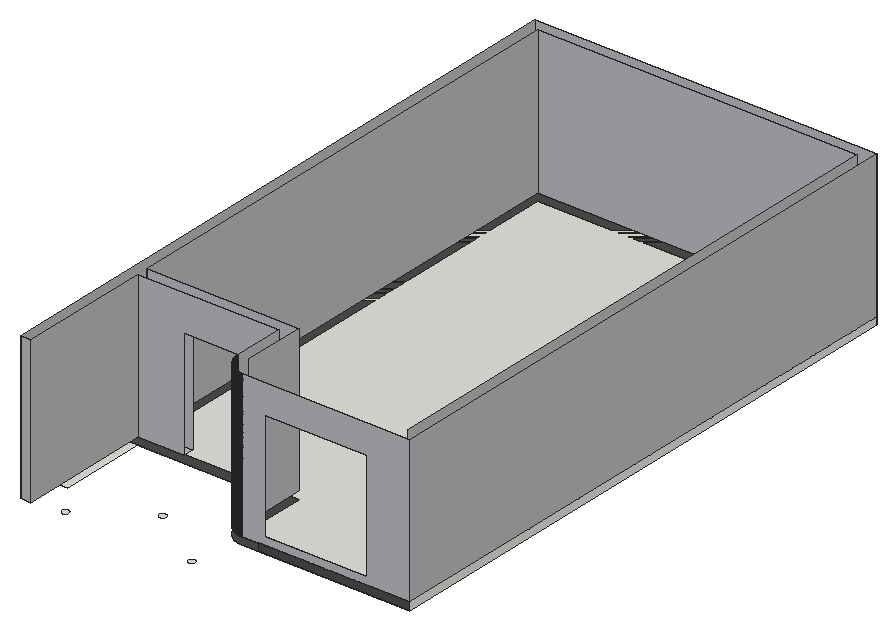
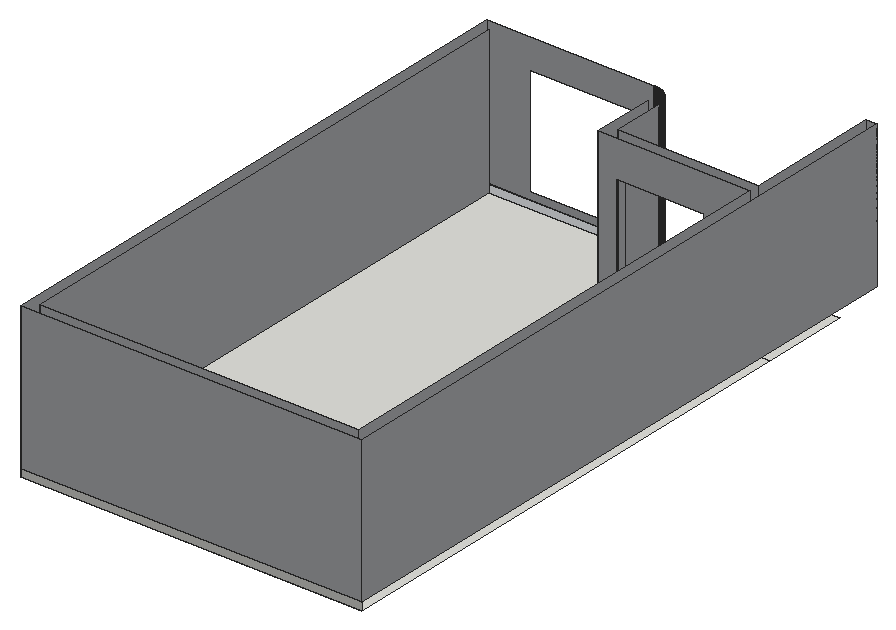
# SketchUp Ruby script. Lengths in inches.
U = 1.inch
M = Sketchup.active_model
def pt(a) = Geom::Point3d.new(a.map { |v| v * U })
def face(e, loops, mat)
  f = e.add_face(loops[0].map { |a| pt(a) })
  loops[1..].each { |l| e.add_face(l.map { |a| pt(a) }).erase! }
  f.material = f.back_material = mat if mat
  f
end
# faces: each face lists its corners as indices into pts; further lists are holes
def faces(e, pts, list, mat = nil) = list.each { |f| face(e, (f[0].is_a?(Array) ? f : [f]).map { |l| l.map { |i| pts[i] } }, mat) }
# xy, xz, yz: faces in a plane at the given z, y or x. An outline is a flat list of corners, or four numbers for a rectangle; further outlines are holes
def ring(l) = l.size == 4 ? [[l[0], l[1]], [l[2], l[1]], [l[2], l[3]], [l[0], l[3]]] : l.each_slice(2).to_a
def flat(e, list, mat, &to3) = list.each { |f| face(e, (f[0].is_a?(Array) ? f : [f]).map { |l| ring(l).map { |u, v| to3.(u, v) } }, mat) }
def xy(e, z, list, mat = nil) = flat(e, list, mat) { |x, y| [x, y, z] }
def xz(e, y, list, mat = nil) = flat(e, list, mat) { |x, z| [x, y, z] }
def yz(e, x, list, mat = nil) = flat(e, list, mat) { |y, z| [x, y, z] }
def lines(e, pts, list) = list.each { |a, b| e.add_line(pt(pts[a]), pt(pts[b])) }
# prism: a flat outline (further loops are holes) pulled along v
def prism(e, loops, v, mat = nil)
  f = face(e, loops, mat); d = Geom::Vector3d.new(v.map { |x| x * U })
  f.pushpull(f.normal.samedirection?(d) ? d.length : -d.length)
end
def box(e, o, s, mat = nil) = prism(e, [[o, [o[0] + s[0], o[1], o[2]], [o[0] + s[0], o[1] + s[1], o[2]], [o[0], o[1] + s[1], o[2]]]], [0, 0, s[2]], mat)
def at(x, y, z, deg = 0) = Geom::Transformation.translation(pt([x, y, z])) * Geom::Transformation.rotation(ORIGIN, Z_AXIS, deg.degrees)
def axes(o, x, y, z) = Geom::Transformation.new([*x, 0, *y, 0, *z, 0, *pt(o).to_a, 1])
def part(name) = M.definitions.add(name)
# library, detail: a bought-in or finely detailed component or shape, given as its bounding box
def library(name, o, s) = part(name).tap { |d| box(d.entities, o, s) }
def detail(e, o, s) = box(e.add_group.entities, o, s)
def put(e, d, t, mat = nil) = e.add_instance(d, t).tap { |i| i.material = mat if mat }
def group(e, t, mat = nil) = e.add_group.tap { |g| g.transformation = t; g.material = mat if mat }.entities
root = M.entities
M.materials.add("1423 AP 8230 BENTONITE").color = [77, 75, 77]
M.materials.add("1427 AP 686 ARMOUR-N").color = [184, 186, 189]
xy(root,245,[[35,153.42,34.92,153.43,34.84,153.43,34.76,153.44,34.6875,153.44,34.61,153.46,34.45,153.48,34.38,153.5,34.3,153.52,34.23,153.55,34.15,153.57,34.01,153.63,33.9375,153.66,33.87,153.7,33.8,153.73,33.73,153.77,33.66,153.8125,33.59,153.86,33.53,153.9,33.29,154.1,33.18,154.21,33.07,154.33,33.02,154.39,32.98,154.45,32.93,154.52,32.89,154.58,32.77,154.79,32.68,155,32.65,155.08,32.62,155.15,32.6,155.23,32.58,155.3,32.54,155.46,32.53,155.53,32.52,155.61,32.51,155.6875,32.51,155.77,32.5,155.85,32.5,156,32.51,156.08,32.51,156.16,32.53,156.32,32.54,156.39,32.58,156.55,32.6,156.62,32.62,156.7,32.68,156.84,32.71,156.92,32.77,157.06,32.85,157.2,32.89,157.26,32.93,157.33,32.98,157.39,33.02,157.46,33.07,157.52,33.18,157.64,33.29,157.75,33.53,157.95,33.59,157.99,33.66,158.04,33.8,158.12,33.87,158.15,33.9375,158.1875,34.01,158.22,34.15,158.28,34.23,158.3,34.3,158.33,34.38,158.35,34.45,158.36,34.53,158.38,34.61,158.39,34.6875,158.4,34.76,158.41,34.84,158.42,35.16,158.42,35.24,158.41,35.3125,158.4,35.39,158.39,35.47,158.38,35.55,158.36,35.62,158.35,35.7,158.33,35.77,158.3,35.85,158.28,35.99,158.22,36.06,158.1875,36.14,158.15,36.2,158.12,36.34,158.04,36.41,157.99,36.47,157.95,36.71,157.75,36.82,157.64,36.93,157.52,36.98,157.46,37.02,157.39,37.07,157.33,37.11,157.26,37.15,157.2,37.23,157.06,37.29,156.92,37.32,156.84,37.38,156.7,37.4,156.62,37.42,156.55,37.46,156.39,37.47,156.32,37.5,156.08,37.5,155.77,37.49,155.6875,37.48,155.61,37.47,155.53,37.46,155.46,37.42,155.3,37.4,155.23,37.38,155.15,37.35,155.08,37.32,155,37.23,154.79,37.11,154.58,37.07,154.52,37.02,154.45,36.98,154.39,36.93,154.33,36.82,154.21,36.71,154.1,36.47,153.9,36.41,153.86,36.34,153.8125,36.27,153.77,36.2,153.73,36.06,153.66,35.85,153.57,35.77,153.55,35.7,153.52,35.62,153.5,35.55,153.48,35.39,153.46,35.3125,153.44,35.24,153.44,35.16,153.43,35.08,153.43],[139,153.42,138.92,153.43,138.84,153.43,138.76,153.44,138.6875,153.44,138.61,153.46,138.45,153.48,138.38,153.5,138.3,153.52,138.23,153.55,138.15,153.57,138.01,153.63,137.9375,153.66,137.87,153.7,137.8,153.73,137.73,153.77,137.66,153.8125,137.59,153.86,137.53,153.9,137.29,154.1,137.18,154.21,137.07,154.33,137.02,154.39,136.98,154.45,136.93,154.52,136.89,154.58,136.77,154.79,136.68,155,136.65,155.08,136.62,155.15,136.6,155.23,136.58,155.3,136.54,155.46,136.53,155.53,136.52,155.61,136.51,155.6875,136.5,155.77,136.5,156.08,136.53,156.32,136.54,156.39,136.58,156.55,136.6,156.62,136.62,156.7,136.68,156.84,136.71,156.92,136.77,157.06,136.85,157.2,136.89,157.26,136.93,157.33,136.98,157.39,137.02,157.46,137.07,157.52,137.18,157.64,137.29,157.75,137.53,157.95,137.59,157.99,137.66,158.04,137.8,158.12,137.87,158.15,137.9375,158.1875,138.01,158.22,138.15,158.28,138.23,158.3,138.3,158.33,138.38,158.35,138.45,158.36,138.53,158.38,138.61,158.39,138.6875,158.4,138.76,158.41,138.84,158.42,139.16,158.42,139.24,158.41,139.3125,158.4,139.39,158.39,139.47,158.38,139.55,158.36,139.62,158.35,139.7,158.33,139.77,158.3,139.85,158.28,139.99,158.22,140.0625,158.1875,140.13,158.15,140.2,158.12,140.34,158.04,140.41,157.99,140.47,157.95,140.71,157.75,140.82,157.64,140.93,157.52,140.98,157.46,141.02,157.39,141.07,157.33,141.11,157.26,141.15,157.2,141.23,157.06,141.29,156.92,141.32,156.84,141.38,156.7,141.4,156.62,141.42,156.55,141.46,156.39,141.47,156.32,141.5,156.08,141.5,155.77,141.49,155.6875,141.48,155.61,141.47,155.53,141.46,155.46,141.42,155.3,141.4,155.23,141.38,155.15,141.35,155.08,141.32,155,141.23,154.79,141.11,154.58,141.07,154.52,141.02,154.45,140.98,154.39,140.93,154.33,140.82,154.21,140.71,154.1,140.47,153.9,140.41,153.86,140.34,153.8125,140.27,153.77,140.2,153.73,140.13,153.7,140.0625,153.66,139.99,153.63,139.85,153.57,139.77,153.55,139.7,153.52,139.62,153.5,139.55,153.48,139.39,153.46,139.3125,153.44,139.24,153.44,139.16,153.43,139.08,153.43],[86.84,188.5,86.76,188.51,86.6875,188.52,86.61,188.53,86.53,188.54,86.45,188.56,86.38,188.58,86.3,188.6,86.23,188.62,86.15,188.65,86.01,188.71,85.9375,188.74,85.87,188.77,85.59,188.93,85.53,188.98,85.47,189.02,85.41,189.07,85.29,189.18,85.23,189.23,85.18,189.29,85.07,189.41,85.02,189.47,84.98,189.53,84.93,189.59,84.77,189.87,84.74,189.9375,84.71,190.01,84.65,190.15,84.62,190.23,84.6,190.3,84.58,190.38,84.56,190.45,84.54,190.53,84.53,190.61,84.52,190.6875,84.51,190.76,84.5,190.84,84.5,191.16,84.51,191.24,84.52,191.3125,84.53,191.39,84.54,191.47,84.56,191.55,84.58,191.62,84.6,191.7,84.62,191.77,84.65,191.85,84.71,191.99,84.74,192.0625,84.77,192.13,84.93,192.41,84.98,192.47,85.02,192.53,85.07,192.59,85.18,192.71,85.23,192.77,85.29,192.82,85.41,192.93,85.47,192.98,85.53,193.02,85.59,193.07,85.87,193.23,85.9375,193.26,86.01,193.29,86.15,193.35,86.23,193.38,86.3,193.4,86.38,193.42,86.45,193.44,86.53,193.46,86.61,193.47,86.6875,193.48,86.76,193.49,86.84,193.5,87.16,193.5,87.24,193.49,87.3125,193.48,87.39,193.47,87.47,193.46,87.55,193.44,87.62,193.42,87.7,193.4,87.77,193.38,87.85,193.35,87.99,193.29,88.0625,193.26,88.13,193.23,88.41,193.07,88.47,193.02,88.53,192.98,88.59,192.93,88.71,192.82,88.77,192.77,88.82,192.71,88.93,192.59,88.98,192.53,89.02,192.47,89.07,192.41,89.23,192.13,89.26,192.0625,89.29,191.99,89.35,191.85,89.38,191.77,89.4,191.7,89.42,191.62,89.44,191.55,89.46,191.47,89.47,191.39,89.48,191.3125,89.49,191.24,89.5,191.16,89.5,190.84,89.49,190.76,89.48,190.6875,89.47,190.61,89.46,190.53,89.44,190.45,89.42,190.38,89.4,190.3,89.38,190.23,89.35,190.15,89.29,190.01,89.26,189.9375,89.23,189.87,89.07,189.59,89.02,189.53,88.98,189.47,88.93,189.41,88.82,189.29,88.77,189.23,88.71,189.18,88.59,189.07,88.53,189.02,88.47,188.98,88.41,188.93,88.13,188.77,88.0625,188.74,87.99,188.71,87.85,188.65,87.77,188.62,87.7,188.6,87.62,188.58,87.55,188.56,87.47,188.54,87.39,188.53,87.3125,188.52,87.24,188.51,87.16,188.5]])
xy(root,246,[[9,180,18,252],[151.78,192,151.57,192.01,151.35,192.01,150.91,192.03,150.7,192.05,150.48,192.0625,150.26,192.08,150.05,192.11,149.83,192.13,149.61,192.16,149.4,192.1875,149.18,192.22,148.97,192.26,148.76,192.29,148.54,192.34,148.12,192.42,147.9,192.47,147.69,192.52,147.48,192.58,147.27,192.63,147.0625,192.69,146.85,192.75,146.64,192.81,146.4375,192.88,146.23,192.95,146.03,193.02,145.82,193.09,145.62,193.17,145.41,193.25,145.01,193.41,144.8125,193.5,144.61,193.59,144.41,193.68,144.22,193.77,144.02,193.86,143.83,193.96,143.63,194.0625,143.44,194.16,143.25,194.27,142.875,194.48,142.6875,194.6,142.5,194.71,142.32,194.83,142.14,194.94,141.95,195.0625,141.77,195.1875,141.6,195.3125,141.42,195.4375,141.24,195.57,140.9,195.83,140.73,195.97,140.56,196.1,140.39,196.24,140.23,196.38,140.0625,196.53,139.9,196.67,139.58,196.97,139.43,197.12,139.27,197.27,139.12,197.43,138.97,197.58,138.67,197.9,138.53,198.0625,138.38,198.23,138.24,198.39,138.1,198.56,137.97,198.73,137.83,198.9,137.57,199.24,137.4375,199.42,137.3125,199.6,137.1875,199.77,137.0625,199.95,136.94,200.14,136.83,200.32,136.71,200.5,136.6,200.6875,136.48,200.875,136.27,201.25,136.16,201.44,136.0625,201.63,135.96,201.83,135.86,202.02,135.77,202.22,135.68,202.41,135.59,202.61,135.5,202.8125,135.41,203.01,135.25,203.41,135.17,203.62,135.09,203.82,135.02,204.03,134.95,204.23,134.88,204.4375,134.81,204.64,134.75,204.85,134.69,205.0625,134.63,205.27,134.58,205.48,134.52,205.69,134.47,205.9,134.42,206.12,134.34,206.54,134.29,206.76,134.26,206.97,134.22,207.18,134.1875,207.4,134.16,207.61,134.13,207.83,134.11,208.05,134.08,208.26,134.0625,208.48,134.05,208.7,134.03,208.91,134.01,209.35,134.01,209.57,134,209.78,134,252,9,252,9,672,290,672,290,192]])
xy(root,246,[[[9,180,18,180,18,252,134,252,134,209.78,134.01,209.57,134.01,209.35,134.03,208.91,134.05,208.7,134.0625,208.48,134.08,208.26,134.11,208.05,134.13,207.83,134.16,207.61,134.1875,207.4,134.22,207.18,134.26,206.97,134.29,206.76,134.34,206.54,134.42,206.12,134.47,205.9,134.52,205.69,134.58,205.48,134.63,205.27,134.69,205.0625,134.75,204.85,134.82,204.64,134.88,204.4375,134.95,204.23,135.02,204.03,135.09,203.82,135.17,203.62,135.25,203.41,135.41,203.01,135.5,202.8125,135.59,202.61,135.68,202.41,135.77,202.22,135.86,202.02,135.96,201.83,136.0625,201.63,136.16,201.44,136.27,201.25,136.48,200.875,136.6,200.6875,136.71,200.5,136.83,200.32,136.94,200.14,137.0625,199.95,137.1875,199.77,137.3125,199.6,137.4375,199.42,137.57,199.24,137.83,198.9,137.97,198.73,138.1,198.56,138.24,198.39,138.38,198.23,138.53,198.0625,138.67,197.9,138.97,197.58,139.12,197.43,139.27,197.27,139.43,197.12,139.58,196.97,139.9,196.67,140.0625,196.53,140.23,196.38,140.39,196.24,140.56,196.1,140.73,195.97,140.9,195.83,141.24,195.57,141.42,195.4375,141.6,195.3125,141.77,195.1875,141.95,195.0625,142.14,194.94,142.32,194.83,142.5,194.71,142.6875,194.6,142.875,194.48,143.25,194.27,143.44,194.16,143.63,194.0625,143.83,193.96,144.02,193.86,144.22,193.77,144.41,193.68,144.61,193.59,144.8125,193.5,145.01,193.41,145.41,193.25,145.62,193.17,145.82,193.09,146.03,193.02,146.23,192.95,146.4375,192.88,146.64,192.82,146.85,192.75,147.0625,192.69,147.27,192.63,147.48,192.58,147.69,192.52,147.9,192.47,148.12,192.42,148.54,192.34,148.76,192.29,148.97,192.26,149.18,192.22,149.4,192.1875,149.61,192.16,149.83,192.13,150.05,192.11,150.26,192.08,150.48,192.0625,150.7,192.05,150.91,192.03,151.35,192.01,151.57,192.01,151.78,192,290,192,290,672,9,672],[151.78,201,151.67,201.01,151.57,201.01,151.46,201.02,151.35,201.02,151.02,201.05,150.92,201.07,150.7,201.09,150.48,201.13,150.38,201.15,150.27,201.17,150.16,201.1875,150.06,201.21,149.95,201.24,149.85,201.26,149.74,201.29,149.64,201.32,149.53,201.35,149.43,201.375,149.32,201.41,149.12,201.47,149.01,201.51,148.91,201.55,148.81,201.58,148.71,201.625,148.61,201.66,148.51,201.71,148.31,201.79,148.21,201.84,148.11,201.88,147.91,201.98,147.82,202.03,147.72,202.08,147.625,202.13,147.53,202.1875,147.4375,202.24,147.34,202.3,147.25,202.35,146.89,202.59,146.8,202.66,146.62,202.78,146.54,202.85,146.45,202.92,146.36,202.98,146.2,203.12,146.11,203.19,146.03,203.26,145.95,203.34,145.79,203.48,145.71,203.56,145.64,203.64,145.56,203.71,145.48,203.79,145.34,203.95,145.26,204.03,145.19,204.11,145.12,204.2,144.98,204.36,144.92,204.45,144.85,204.54,144.78,204.62,144.66,204.8,144.59,204.89,144.35,205.25,144.3,205.34,144.24,205.4375,144.1875,205.53,144.13,205.625,144.08,205.72,144.03,205.82,143.98,205.91,143.88,206.11,143.84,206.21,143.79,206.31,143.71,206.51,143.66,206.61,143.625,206.71,143.58,206.81,143.55,206.91,143.51,207.01,143.47,207.12,143.41,207.32,143.375,207.43,143.35,207.53,143.32,207.64,143.29,207.74,143.26,207.85,143.24,207.95,143.21,208.06,143.1875,208.16,143.17,208.27,143.15,208.38,143.13,208.48,143.09,208.7,143.07,208.92,143.05,209.02,143.02,209.35,143.02,209.46,143.01,209.57,143.01,209.67,143,209.78,143,261,18,261,18,663,281,663,281,201]]],"1423 AP 8230 BENTONITE")
xy(root,252,[[9,141.92,9,672,290,672,290,192,151.78,192,151.57,192.01,151.35,192.01,150.91,192.03,150.7,192.05,150.48,192.0625,150.26,192.08,150.05,192.11,149.83,192.13,149.61,192.16,149.4,192.1875,149.18,192.22,148.97,192.26,148.76,192.29,148.54,192.34,148.12,192.42,147.9,192.47,147.69,192.52,147.48,192.58,147.27,192.63,147.0625,192.69,146.85,192.75,146.64,192.82,146.4375,192.88,146.23,192.95,146.03,193.02,145.82,193.09,145.62,193.17,145.41,193.25,145.01,193.41,144.8125,193.5,144.61,193.59,144.41,193.68,144.22,193.77,144.02,193.86,143.83,193.96,143.63,194.0625,143.44,194.16,143.25,194.27,142.875,194.48,142.6875,194.6,142.5,194.71,142.32,194.83,142.14,194.94,141.95,195.0625,141.77,195.1875,141.6,195.3125,141.42,195.4375,141.24,195.57,140.9,195.83,140.73,195.97,140.56,196.1,140.39,196.24,140.23,196.38,140.0625,196.53,139.9,196.67,139.58,196.97,139.43,197.12,139.27,197.27,139.12,197.43,138.97,197.58,138.67,197.9,138.53,198.0625,138.38,198.23,138.24,198.39,138.1,198.56,137.97,198.73,137.83,198.9,137.57,199.24,137.4375,199.42,137.3125,199.6,137.1875,199.77,137.0625,199.95,136.94,200.14,136.83,200.32,136.71,200.5,136.6,200.6875,136.48,200.875,136.27,201.25,136.16,201.44,136.0625,201.63,135.96,201.83,135.86,202.02,135.77,202.22,135.68,202.41,135.59,202.61,135.5,202.8125,135.41,203.01,135.25,203.41,135.17,203.62,135.09,203.82,135.02,204.03,134.95,204.23,134.88,204.4375,134.82,204.64,134.75,204.85,134.69,205.0625,134.63,205.27,134.58,205.48,134.52,205.69,134.47,205.9,134.42,206.12,134.34,206.54,134.29,206.76,134.26,206.97,134.22,207.18,134.1875,207.4,134.16,207.61,134.13,207.83,134.11,208.05,134.08,208.26,134.0625,208.48,134.05,208.7,134.03,208.91,134.01,209.35,134.01,209.57,134,209.78,134,252,128,252,128,261,143,261,143,209.78,143.01,209.67,143.01,209.57,143.02,209.46,143.02,209.35,143.05,209.02,143.07,208.92,143.09,208.7,143.13,208.48,143.15,208.38,143.17,208.27,143.1875,208.16,143.21,208.06,143.24,207.95,143.26,207.85,143.29,207.74,143.32,207.64,143.35,207.53,143.375,207.43,143.41,207.32,143.47,207.12,143.51,207.01,143.55,206.91,143.58,206.81,143.625,206.71,143.66,206.61,143.71,206.51,143.79,206.31,143.84,206.21,143.88,206.11,143.98,205.91,144.03,205.82,144.08,205.72,144.13,205.625,144.1875,205.53,144.24,205.4375,144.3,205.34,144.35,205.25,144.59,204.89,144.66,204.8,144.78,204.62,144.85,204.54,144.92,204.45,144.98,204.36,145.12,204.2,145.19,204.11,145.26,204.03,145.34,203.95,145.48,203.79,145.56,203.71,145.64,203.64,145.71,203.56,145.79,203.48,145.95,203.34,146.03,203.26,146.11,203.19,146.2,203.12,146.36,202.98,146.45,202.92,146.54,202.85,146.62,202.78,146.8,202.66,146.89,202.59,147.25,202.35,147.34,202.3,147.4375,202.24,147.53,202.1875,147.625,202.13,147.72,202.08,147.82,202.03,147.91,201.98,148.11,201.88,148.21,201.84,148.31,201.79,148.51,201.71,148.61,201.66,148.71,201.625,148.81,201.58,148.91,201.55,149.01,201.51,149.12,201.47,149.32,201.41,149.43,201.375,149.53,201.35,149.64,201.32,149.74,201.29,149.85,201.26,149.95,201.24,150.06,201.21,150.16,201.1875,150.27,201.17,150.38,201.15,150.48,201.13,150.7,201.09,150.92,201.07,151.02,201.05,151.35,201.02,151.46,201.02,151.57,201.01,151.67,201.01,151.78,201,281,201,281,663,18,663,18,261,56,261,56,252,18,252,18,141.92]],"1427 AP 686 ARMOUR-N")
xz(root,141.92,[[9,252,18,372]],"1427 AP 686 ARMOUR-N")
xz(root,192,[[165,246,290,252]],"1423 AP 8230 BENTONITE")
xz(root,192,[[151.78,252,152,372],[[152,252,290,372],[170,258,254,348]]],"1427 AP 686 ARMOUR-N")
xz(root,192.01,[[151.35,252,151.57,372]],"1427 AP 686 ARMOUR-N")
xz(root,252,[[18,252,56,252,56,342,128,342,128,252,134,252,134,372,18,372]],"1427 AP 686 ARMOUR-N")
xz(root,261,[[18,252,18,372,143,372,143,252,128,252,128,342,56,342,56,252]],"1427 AP 686 ARMOUR-N")
xz(root,663,[[18,252,281,372]],"1427 AP 686 ARMOUR-N")
xz(root,672,[[9,246,290,252]])
xz(root,672,[[9,252,290,372]],"1427 AP 686 ARMOUR-N")
yz(root,9,[[141.92,252,672,372]],"1427 AP 686 ARMOUR-N")
yz(root,18,[[141.92,252,252,372],[261,252,663,372]],"1427 AP 686 ARMOUR-N")
yz(root,134,[[210,252,252,372]],"1427 AP 686 ARMOUR-N")
yz(root,143,[[209.89,252,261,372]],"1427 AP 686 ARMOUR-N")
yz(root,281,[[201,252,663,372]],"1427 AP 686 ARMOUR-N")
yz(root,290,[[192,246,672,252]])
yz(root,290,[[192,252,672,372]],"1427 AP 686 ARMOUR-N")
p = [[150.7,192.05,372],[150.48,192.0625,372],[150.48,192.0625,252],[150.7,192.05,252],[150.91,192.03,372],[150.91,192.03,252],
  [151.13,192.02,372],[151.13,192.02,252],[151.35,192.01,372],[151.35,192.01,252],[151.78,192,372],[151.57,192.01,372],
  [151.57,192.01,252],[151.78,192,252],[149.83,192.13,372],[149.61,192.16,372],[149.61,192.16,252],[149.83,192.13,252],
  [150.05,192.11,372],[150.05,192.11,252],[150.26,192.08,372],[150.26,192.08,252],[149.18,192.22,372],[148.97,192.26,372],
  [148.97,192.26,252],[149.18,192.22,252],[149.4,192.1875,372],[149.4,192.1875,252],[148.54,192.34,372],[148.33,192.38,372],
  [148.33,192.38,252],[148.54,192.34,252],[148.76,192.29,372],[148.76,192.29,252],[148.12,192.42,372],[147.9,192.47,372],
  [147.9,192.47,252],[148.12,192.42,252],[147.69,192.52,372],[147.48,192.58,372],[147.48,192.58,252],[147.69,192.52,252],
  [147.27,192.63,372],[147.0625,192.69,372],[147.0625,192.69,252],[147.27,192.63,252],[146.85,192.75,372],[146.85,192.75,252],
  [146.64,192.82,372],[146.4375,192.88,372],[146.4375,192.88,252],[146.64,192.82,252],[146.23,192.95,372],[146.03,193.02,372],
  [146.03,193.02,252],[146.23,192.95,252],[145.82,193.09,372],[145.82,193.09,252],[145.62,193.17,372],[145.62,193.17,252],
  [145.41,193.25,372],[145.21,193.33,372],[145.21,193.33,252],[145.41,193.25,252],[145.01,193.41,372],[145.01,193.41,252],
  [144.8125,193.5,372],[144.8125,193.5,252],[144.61,193.59,372],[144.61,193.59,252],[144.41,193.68,372],[144.41,193.68,252],
  [144.22,193.77,372],[144.22,193.77,252],[144.02,193.86,372],[144.02,193.86,252],[143.83,193.96,372],[143.83,193.96,252],
  [143.63,194.0625,372],[143.63,194.0625,252],[143.44,194.16,372],[143.44,194.16,252],[143.25,194.27,372],[143.25,194.27,252],
  [143.0625,194.375,372],[143.0625,194.375,252],[142.875,194.48,372],[142.875,194.48,252],[142.6875,194.6,372],[142.6875,194.6,252],
  [142.5,194.71,372],[142.5,194.71,252],[142.32,194.83,372],[142.32,194.83,252],[142.14,194.94,372],[142.14,194.94,252],
  [141.95,195.0625,372],[141.95,195.0625,252],[141.77,195.1875,372],[141.77,195.1875,252],[141.6,195.3125,372],[141.6,195.3125,252],
  [141.42,195.4375,372],[141.42,195.4375,252],[141.24,195.57,372],[141.24,195.57,252],[141.07,195.7,372],[141.07,195.7,252],
  [140.9,195.83,372],[140.9,195.83,252],[140.73,195.97,372],[140.73,195.97,252],[140.56,196.1,372],[140.56,196.1,252],
  [140.39,196.24,372],[140.39,196.24,252],[140.23,196.38,372],[140.23,196.38,252],[140.0625,196.53,372],[140.0625,196.53,252],
  [139.9,196.67,372],[139.9,196.67,252],[139.74,196.82,372],[139.74,196.82,252],[139.58,196.97,372],[139.58,196.97,252],
  [139.43,197.12,372],[139.43,197.12,252],[139.27,197.27,372],[139.27,197.27,252],[139.12,197.43,372],[139.12,197.43,252],
  [138.97,197.58,372],[138.97,197.58,252],[138.82,197.74,372],[138.82,197.74,252],[138.67,197.9,372],[138.67,197.9,252],
  [138.53,198.0625,372],[138.53,198.0625,252],[138.38,198.23,372],[138.38,198.23,252],[138.24,198.39,372],[138.24,198.39,252],
  [138.1,198.56,372],[138.1,198.56,252],[137.97,198.73,372],[137.97,198.73,252],[137.83,198.9,372],[137.83,198.9,252],
  [137.7,199.07,372],[137.7,199.07,252],[137.57,199.24,372],[137.57,199.24,252],[137.4375,199.42,372],[137.4375,199.42,252],
  [137.3125,199.6,372],[137.3125,199.6,252],[137.1875,199.77,372],[137.1875,199.77,252],[137.0625,199.95,372],[137.0625,199.95,252],
  [136.94,200.14,372],[136.94,200.14,252],[136.83,200.32,372],[136.83,200.32,252],[136.71,200.5,372],[136.71,200.5,252],
  [136.6,200.6875,372],[136.6,200.6875,252],[136.48,200.875,372],[136.48,200.875,252],[136.375,201.0625,372],[136.375,201.0625,252],
  [136.27,201.25,372],[136.27,201.25,252],[136.16,201.44,372],[136.16,201.44,252],[136.0625,201.63,372],[136.0625,201.63,252],
  [135.96,201.83,372],[135.96,201.83,252],[135.86,202.02,372],[135.86,202.02,252],[135.77,202.22,372],[135.77,202.22,252],
  [135.68,202.41,372],[135.68,202.41,252],[135.59,202.61,372],[135.59,202.61,252],[135.5,202.8125,372],[135.5,202.8125,252],
  [135.41,203.01,372],[135.41,203.01,252],[135.33,203.21,372],[135.33,203.21,252],[135.25,203.41,372],[135.25,203.41,252],
  [135.17,203.62,372],[135.17,203.62,252],[135.09,203.82,372],[135.09,203.82,252],[135.02,204.03,372],[135.02,204.03,252],
  [134.95,204.23,372],[134.95,204.23,252],[134.88,204.4375,372],[134.88,204.4375,252],[134.82,204.64,372],[134.82,204.64,252],
  [134.75,204.85,372],[134.75,204.85,252],[134.69,205.0625,372],[134.69,205.0625,252],[134.63,205.27,372],[134.63,205.27,252],
  [134.58,205.48,372],[134.58,205.48,252],[134.52,205.69,372],[134.52,205.69,252],[134.47,205.9,372],[134.47,205.9,252],
  [134.42,206.12,372],[134.42,206.12,252],[134.38,206.33,372],[134.38,206.33,252],[134.34,206.54,372],[134.34,206.54,252],
  [134.29,206.76,372],[134.29,206.76,252],[134.26,206.97,372],[134.26,206.97,252],[134.22,207.18,372],[134.22,207.18,252],
  [134.1875,207.4,372],[134.1875,207.4,252],[134.16,207.61,372],[134.16,207.61,252],[134.13,207.83,372],[134.13,207.83,252],
  [134.11,208.05,372],[134.11,208.05,252],[134.08,208.26,372],[134.08,208.26,252],[134.0625,208.48,372],[134.0625,208.48,252],
  [134.05,208.7,372],[134.05,208.7,252],[134.03,208.91,372],[134.03,208.91,252],[134.02,209.13,372],[134.02,209.13,252],
  [134.01,209.35,372],[134.01,209.35,252],[151.97,192,252],[151.97,192,246],[134,209.97,252],[134,209.97,246],
  [134,208.09,246]]
faces(root,p,[[0,1,2,3],[4,0,3,5],[6,4,5,7],[8,6,7,9],[10,11,12,13],[14,15,16,17],[18,14,17,19],[20,18,19,21],
  [1,20,21,2],[22,23,24,25],[26,22,25,27],[15,26,27,16],[28,29,30,31],[32,28,31,33],[23,32,33,24],[34,35,36,37],
  [29,34,37,30],[38,39,40,41],[35,38,41,36],[42,43,44,45],[39,42,45,40],[43,46,47,44],[48,49,50,51],[46,48,51,47],
  [52,53,54,55],[49,52,55,50],[53,56,57,54],[56,58,59,57],[60,61,62,63],[58,60,63,59],[61,64,65,62],[64,66,67,65],
  [66,68,69,67],[68,70,71,69],[70,72,73,71],[72,74,75,73],[74,76,77,75],[76,78,79,77],[78,80,81,79],[80,82,83,81],
  [82,84,85,83],[84,86,87,85],[86,88,89,87],[88,90,91,89],[90,92,93,91],[92,94,95,93],[94,96,97,95],[96,98,99,97],
  [98,100,101,99],[100,102,103,101],[102,104,105,103],[104,106,107,105],[106,108,109,107],[108,110,111,109],[110,112,113,111],[112,114,115,113],
  [114,116,117,115],[116,118,119,117],[118,120,121,119],[120,122,123,121],[122,124,125,123],[124,126,127,125],[126,128,129,127],[128,130,131,129],
  [130,132,133,131],[132,134,135,133],[134,136,137,135],[136,138,139,137],[138,140,141,139],[140,142,143,141],[142,144,145,143],[144,146,147,145],
  [146,148,149,147],[148,150,151,149],[150,152,153,151],[152,154,155,153],[154,156,157,155],[156,158,159,157],[158,160,161,159],[160,162,163,161],
  [162,164,165,163],[164,166,167,165],[166,168,169,167],[168,170,171,169],[170,172,173,171],[172,174,175,173],[174,176,177,175],[176,178,179,177],
  [178,180,181,179],[180,182,183,181],[182,184,185,183],[184,186,187,185],[186,188,189,187],[188,190,191,189],[190,192,193,191],[192,194,195,193],
  [194,196,197,195],[196,198,199,197],[198,200,201,199],[200,202,203,201],[202,204,205,203],[204,206,207,205],[206,208,209,207],[208,210,211,209],
  [210,212,213,211],[212,214,215,213],[214,216,217,215],[216,218,219,217],[218,220,221,219],[220,222,223,221],[222,224,225,223],[224,226,227,225],
  [226,228,229,227],[228,230,231,229],[230,232,233,231],[232,234,235,233],[234,236,237,235],[236,238,239,237],[238,240,241,239],[240,242,243,241],
  [242,244,245,243],[244,246,247,245],[246,248,249,247],[248,250,251,249],[250,252,253,251]],"1427 AP 686 ARMOUR-N")
lines(root,p,[[254,255],[256,257],[257,258]])
